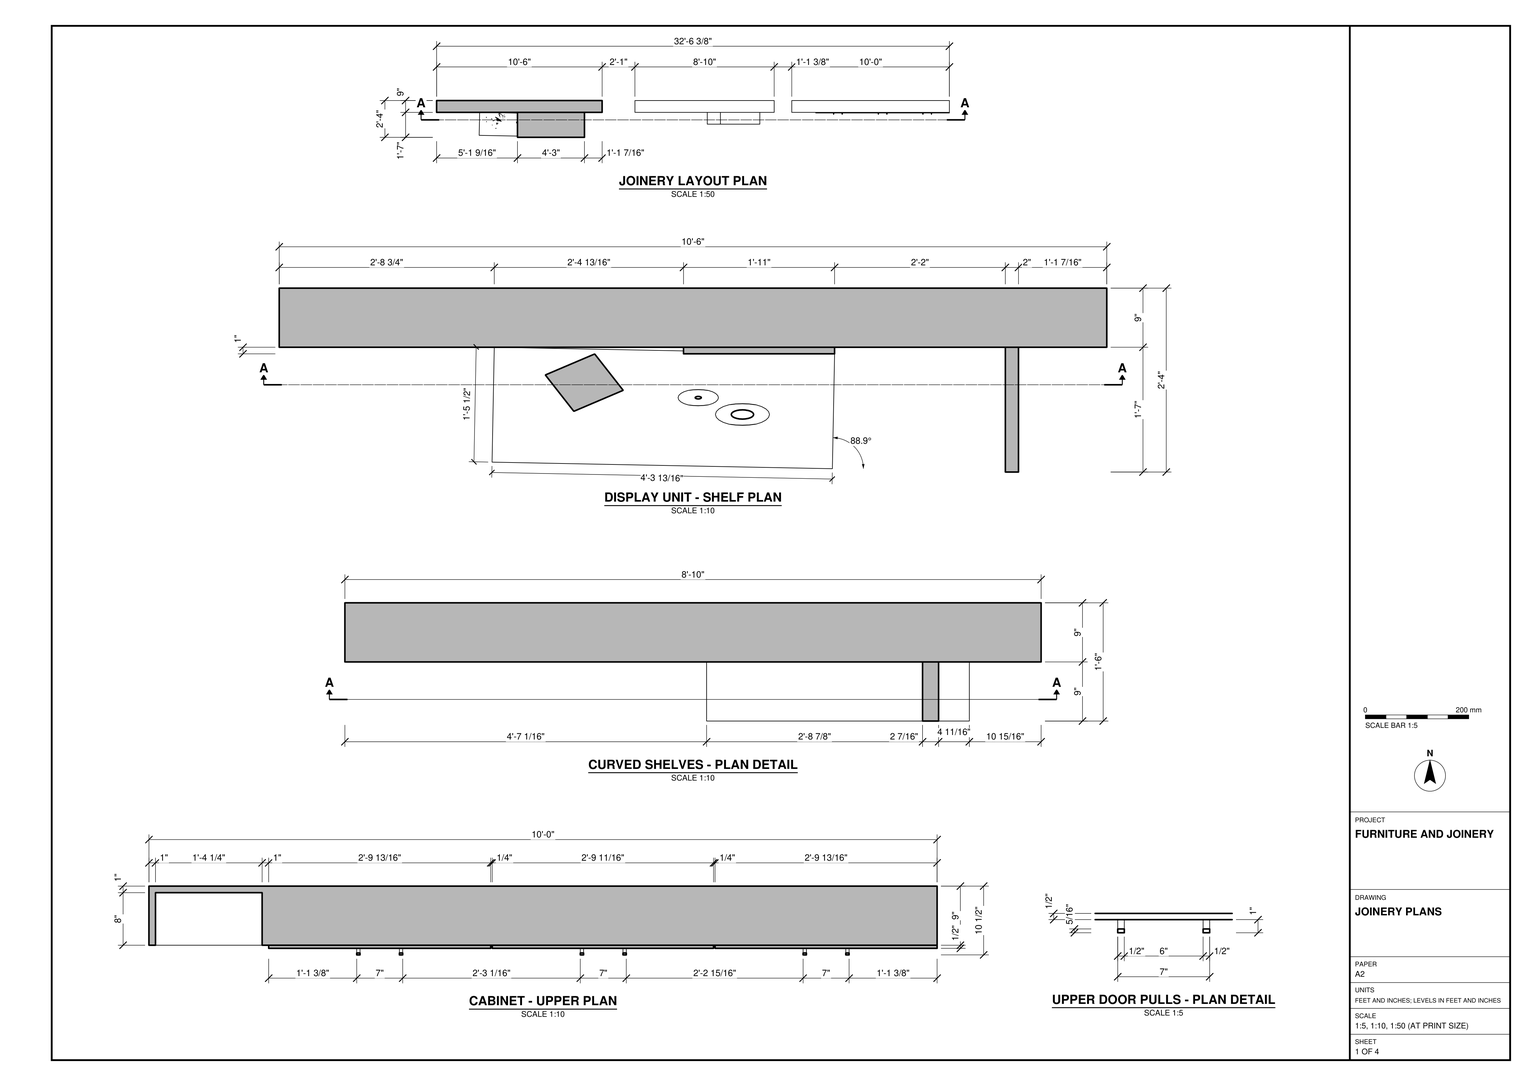
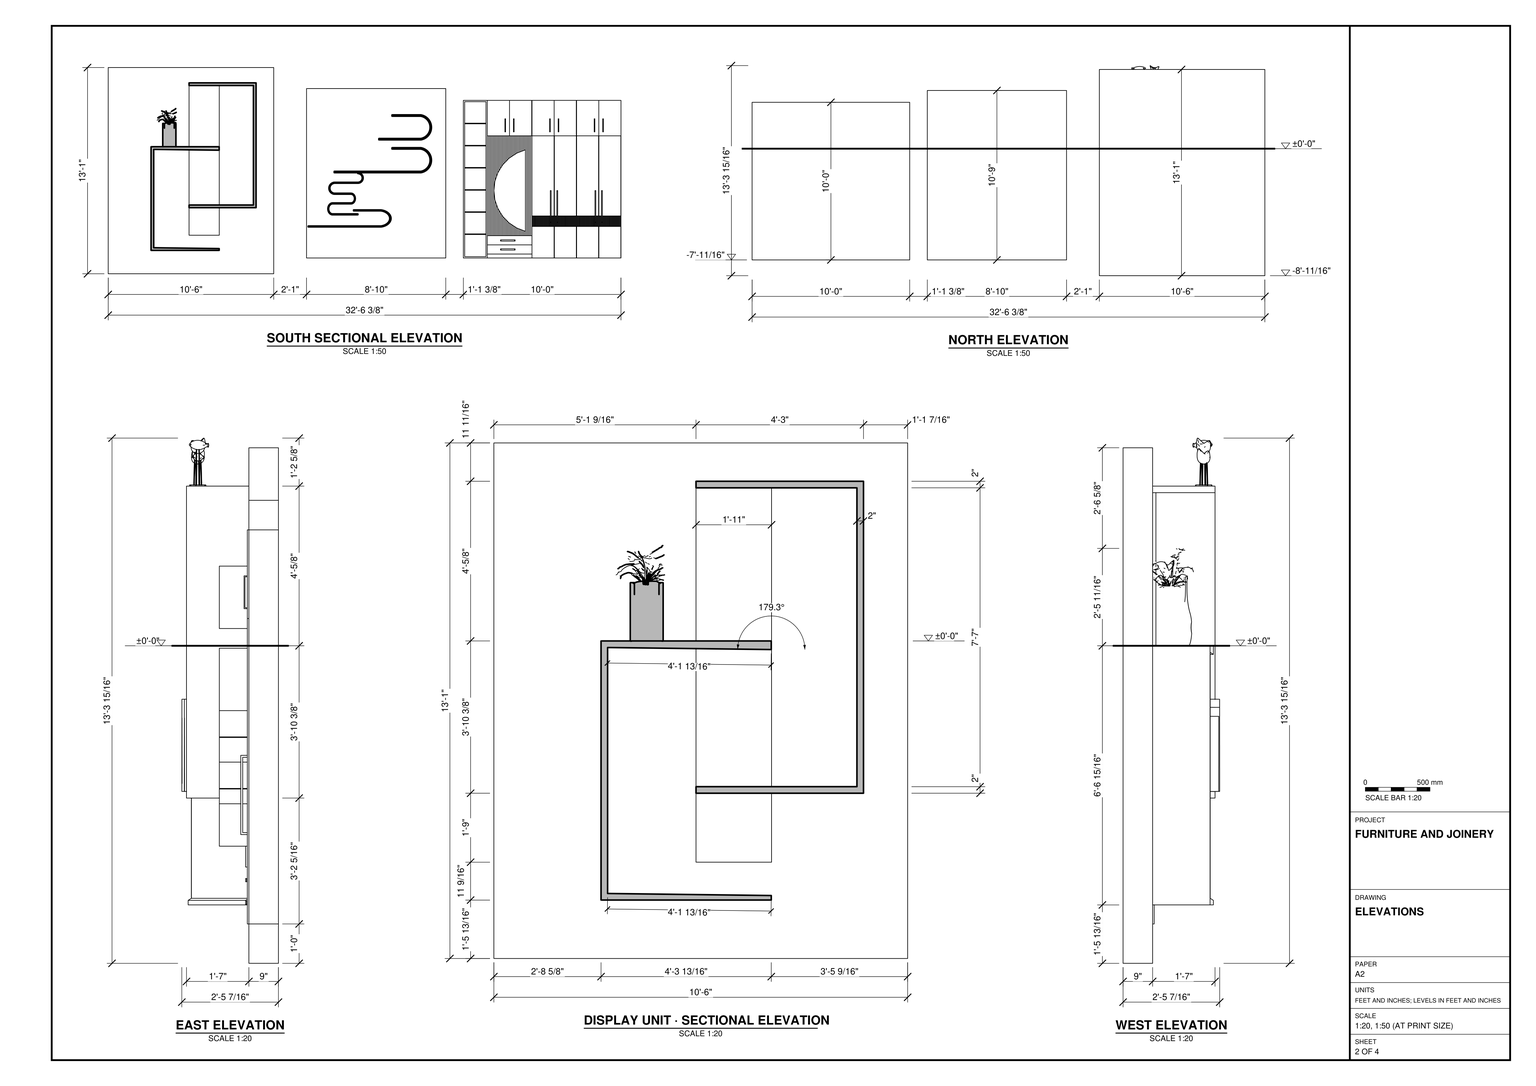
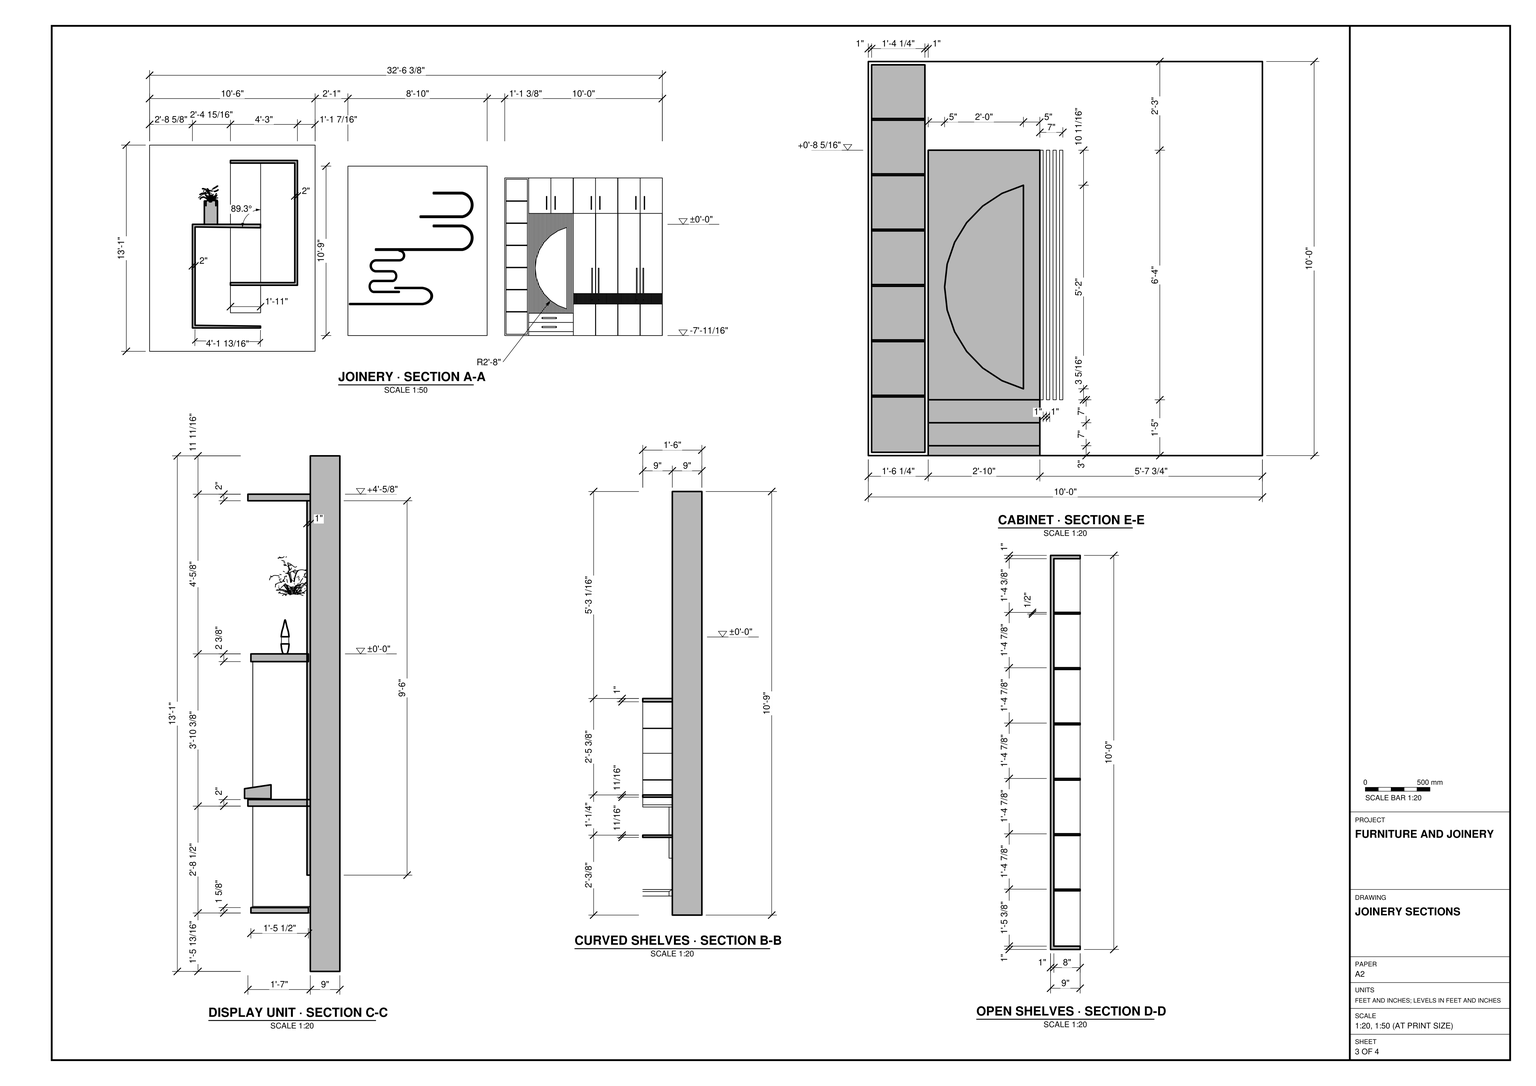
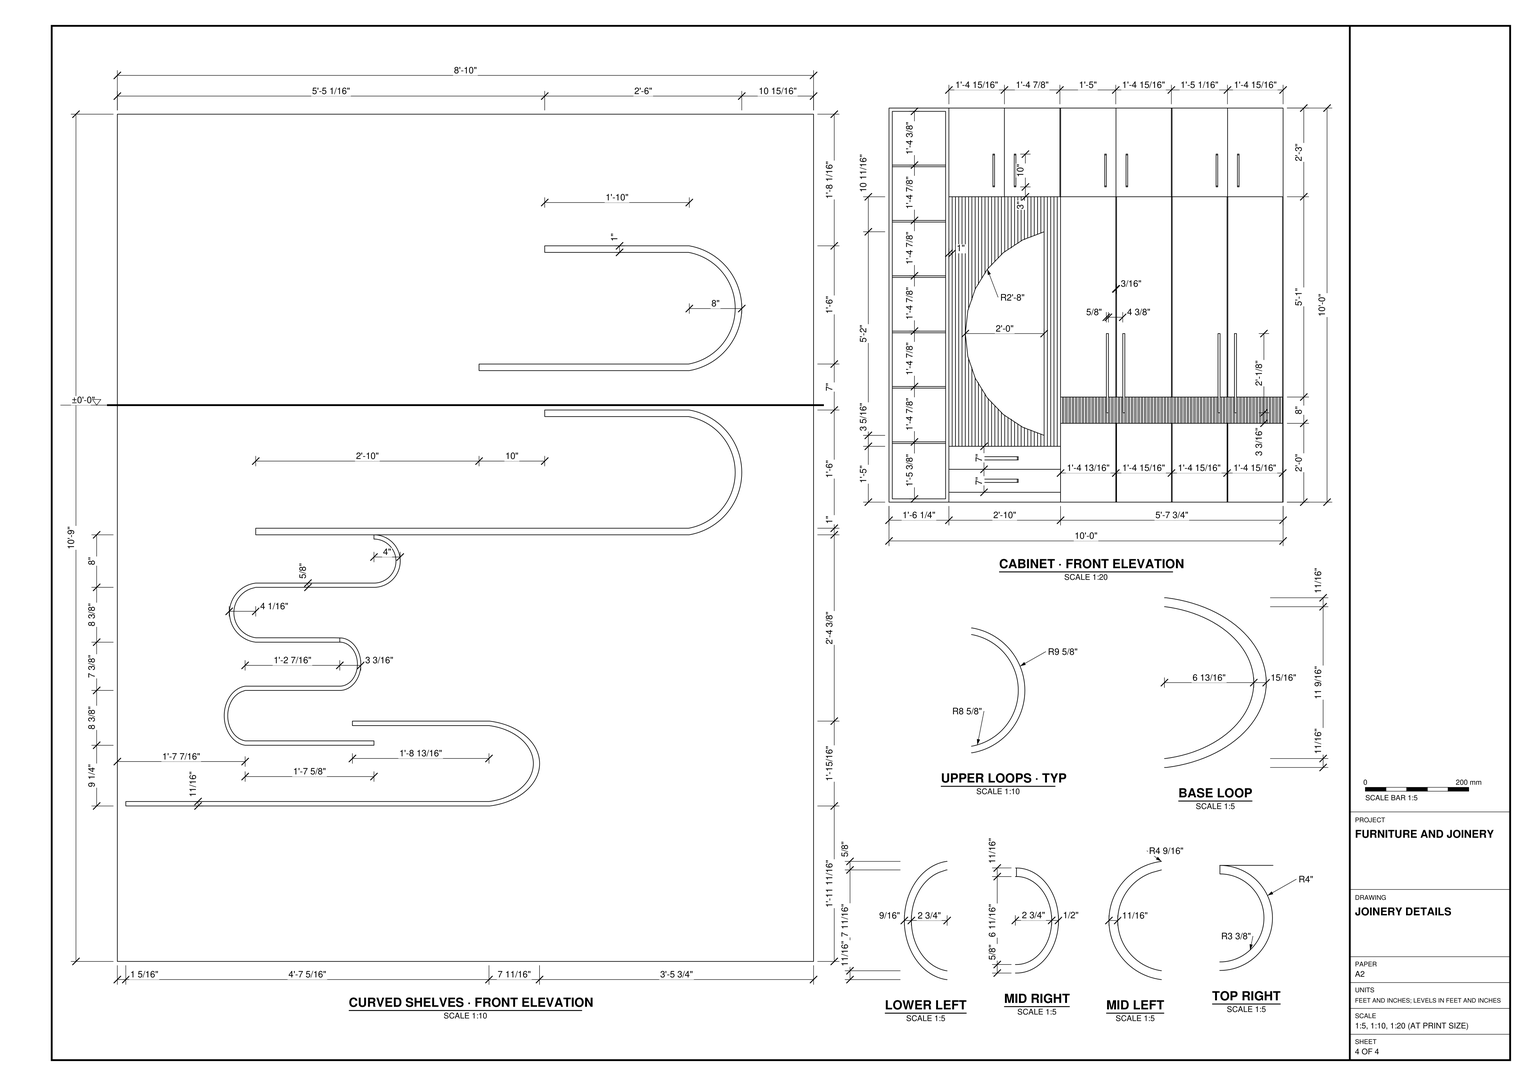
Build the three joinery pieces in SketchUp from task_files/diagram_01.pdf. Work in feet and inches. The complete arrangement is 32'-6 3/8" wide, 2'-5 7/16" deep and 13'-3 15/16" high. Use ±0'-0" as the common elevation datum, not as the bottom of the units.

Follow the south elevation from left to right: the framed display unit, the curved shelves and the storage cabinet. Align their backs in plan and leave the gaps dimensioned on the layout sheet. On the display unit, model the 9" thick backing panel and the projecting shelves with their vertical returns. The lower frame opens to the right and the upper frame opens to the left. On the middle unit, follow the horizontal shelf runs and rounded returns as they rise from the lower left to the upper right. Use the sections to set the shelf projections from the backing panels.

Build the cabinet with a full-height column of open shelves at the left, a recessed display bay with a semicircular feature above two drawers, and closed storage at the right. Include the upper doors, lower fronts and projecting pulls shown in the drawings. Decor and loose items may be any suitable library components placed as shown. Keep each joinery piece in a separate group or component and use components for repeated parts. Save one SketchUp model as output_files/display_unit_curved_shelves_and_storage_cabinet.skp.

# SketchUp Ruby script. Lengths in inches.
U = 1.inch
M = Sketchup.active_model
def pt(a) = Geom::Point3d.new(a.map { |v| v * U })
def face(e, loops, mat)
  f = e.add_face(loops[0].map { |a| pt(a) })
  loops[1..].each { |l| e.add_face(l.map { |a| pt(a) }).erase! }
  f.material = f.back_material = mat if mat
  f
end
# faces: each face lists its corners as indices into pts; further lists are holes
def faces(e, pts, list, mat = nil) = list.each { |f| face(e, (f[0].is_a?(Array) ? f : [f]).map { |l| l.map { |i| pts[i] } }, mat) }
# xy, xz, yz: faces in a plane at the given z, y or x. An outline is a flat list of corners, or four numbers for a rectangle; further outlines are holes
def ring(l) = l.size == 4 ? [[l[0], l[1]], [l[2], l[1]], [l[2], l[3]], [l[0], l[3]]] : l.each_slice(2).to_a
def flat(e, list, mat, &to3) = list.each { |f| face(e, (f[0].is_a?(Array) ? f : [f]).map { |l| ring(l).map { |u, v| to3.(u, v) } }, mat) }
def xy(e, z, list, mat = nil) = flat(e, list, mat) { |x, y| [x, y, z] }
def xz(e, y, list, mat = nil) = flat(e, list, mat) { |x, z| [x, y, z] }
def yz(e, x, list, mat = nil) = flat(e, list, mat) { |y, z| [x, y, z] }
def lines(e, pts, list) = list.each { |a, b| e.add_line(pt(pts[a]), pt(pts[b])) }
# prism: a flat outline (further loops are holes) pulled along v
def prism(e, loops, v, mat = nil)
  f = face(e, loops, mat); d = Geom::Vector3d.new(v.map { |x| x * U })
  f.pushpull(f.normal.samedirection?(d) ? d.length : -d.length)
end
def box(e, o, s, mat = nil) = prism(e, [[o, [o[0] + s[0], o[1], o[2]], [o[0] + s[0], o[1] + s[1], o[2]], [o[0], o[1] + s[1], o[2]]]], [0, 0, s[2]], mat)
def at(x, y, z, deg = 0) = Geom::Transformation.translation(pt([x, y, z])) * Geom::Transformation.rotation(ORIGIN, Z_AXIS, deg.degrees)
def axes(o, x, y, z) = Geom::Transformation.new([*x, 0, *y, 0, *z, 0, *pt(o).to_a, 1])
def part(name) = M.definitions.add(name)
# library, detail: a bought-in or finely detailed component or shape, given as its bounding box
def library(name, o, s) = part(name).tap { |d| box(d.entities, o, s) }
def detail(e, o, s) = box(e.add_group.entities, o, s)
def put(e, d, t, mat = nil) = e.add_instance(d, t).tap { |i| i.material = mat if mat }
def group(e, t, mat = nil) = e.add_group.tap { |g| g.transformation = t; g.material = mat if mat }.entities
root = M.entities
M.materials.add("[Color A01]").color = [101, 116, 79]
M.materials.add("[Color A01]1").color = [196, 189, 165]
M.materials.add("[Color A01]2").color = [176, 132, 93]
M.materials.add("[Color A02]").color = [127, 133, 94]
M.materials.add("[Color C02]").color = [255, 204, 153]
M.materials.add("[Color M09]").color = [0, 0, 0]
M.materials.add("[Wood Cherry Original]").color = [152, 86, 42]
c1 = library("Untitled",[0,0,0],[7.78,10.125,9.38])
c2 = library("Ceramic Birds on",[-120.01,56.07,-27.09],[117.74,27.05,54.18])
c3 = library("SimLab\#1",[-237.64,52,0],[43.92,43.98,50.37])
c4 = part("Vertical wood slat")
box(c4.entities,[0,-2,0],[1,2,76],"[Wood Cherry Original]")
c5 = part("Group\#7")
prism(c5.entities,[[[0.625,2,0],[0.625,2,0.59],[0.625,0.59,0.59],[0.625,0.59,23.53],[0.625,2,23.53],[0.625,2,24.13],[0.625,0,24.13],[0.625,0,0]]],[-0.625,0,0])
c6 = part("Group\#5")
prism(c6.entities,[[[0.5,1,9.71],[0.5,1,10],[0.5,0,10],[0.5,0,0],[0.5,1,0],[0.5,1,0.29],[0.5,0.29,0.29],[0.5,0.29,9.71]]],[-0.5,0,0])
c7 = library("Group\#37",[208.35,-82.82,84.7],[13.92,5.45,20.99])
xy(root,5.8,[[84.22,0.51,32.41,1.51,32.74,19,84.56,18]],"[Color A01]2")
xy(root,84.7,[[84.22,0.51,84.56,18,32.74,19,32.41,1.51]],"[Color A01]2")
p = [[84.22,0.51,5.8],[84.22,0.51,7.18],[34.4,1.47,7.8],[34.4,1.47,82.7],[84.22,0.51,82.08],[84.22,0.51,84.7],
  [32.41,1.51,84.7],[32.41,1.51,5.8],[84.56,18,5.8],[84.56,18,7.18],[32.74,19,84.7],[32.74,19,5.8],
  [84.56,18,84.7],[84.56,18,82.08],[34.74,18.96,82.7],[34.74,18.96,7.8]]
faces(root,p,[[0,1,2,3,4,5,6,7],[10,11,7,6],[3,2,15,14],[4,3,14,13],[4,13,12,5]],"[Color A01]2")
faces(root,p,[[8,9,1,0],[12,13,14,15,9,8,11,10]])
put(root,c1,axes([110.34,0.03,40.32],[-0.12671,1.68524,0],[-4.76654,-0.3584,0],[0,0,3]))
put(root,c2,axes([102.2,-15.7,140.64],[0.23902,0,0],[0,0.28,0],[0,0,0.2698]))
put(root,c3,axes([171.33,-17.61,84.65],[0.58,0,0],[0,0.4272,0],[0,0,0.59]))
g1 = group(root,at(270.37,16.53,0))
prism(g1,[[[39.05,2.47,12.84],[39.35,2.47,12.84],[39.35,1.47,12.84],[28.35,1.47,12.84],[28.35,2.47,12.84],[28.65,2.47,12.84],[28.65,1.77,12.84],[39.05,1.77,12.84]]],[0,0,1],"[Color M09]")
prism(g1,[[[39.05,2.47,6],[39.35,2.47,6],[39.35,1.47,6],[28.35,1.47,6],[28.35,2.47,6],[28.65,2.47,6],[28.65,1.77,6],[39.05,1.77,6]]],[0,0,1],"[Color M09]")
put(g1,c4,at(34.23,10.47,17))
put(g1,c4,at(24.23,10.47,17))
put(g1,c4,at(46.23,10.47,17))
put(g1,c4,at(48.23,10.47,17))
put(g1,c4,at(44.23,10.47,17))
put(g1,c4,at(18.23,10.47,17))
put(g1,c4,at(20.23,10.47,17))
put(g1,c4,at(26.23,10.47,17))
put(g1,c4,at(42.23,10.47,17))
put(g1,c4,at(28.23,10.47,17))
put(g1,c4,at(36.23,10.47,17))
put(g1,c4,at(30.23,10.47,17))
put(g1,c4,at(22.23,10.47,17))
put(g1,c4,at(32.23,10.47,17))
put(g1,c4,at(38.23,10.47,17))
put(g1,c4,at(40.23,10.47,17))
put(g1,c4,at(50.23,10.47,17))
put(g1,c4,at(54.23,10.47,17))
put(g1,c4,at(58.23,10.47,17))
put(g1,c4,at(52.23,10.47,17))
put(g1,c4,at(56.23,10.47,17))
g2 = group(g1,at(23.23,8.39,20.33))
xz(g2,0,[[[24,0,17.44,2.49,11.58,6.35,6.7,11.4,3.04,17.38,0.77,24.02,0,31,0.77,37.98,3.04,44.62,6.7,50.6,11.58,55.65,17.44,59.51,24,62],[21.5,3.63,21.5,58.37,18.59,57.27,13.1875,53.71,8.69,49.06,5.32,43.54,3.23,37.43,2.52,31,3.23,24.57,5.32,18.46,8.69,12.94,13.1875,8.29,18.59,4.73]]])
g3 = group(g1,at(23.23,6.31,20.33))
xz(g3,0,[[24,0,24,62,17.44,59.51,11.58,55.65,6.7,50.6,3.04,44.62,0.77,37.98,0,31,0.77,24.02,3.04,17.38,6.7,11.4,11.58,6.35,17.44,2.49]])
xz(g3,2,[[[24,0,17.44,2.49,11.58,6.35,6.7,11.4,3.04,17.38,0.77,24.02,0,31,0.77,37.98,3.04,44.62,6.7,50.6,11.58,55.65,17.44,59.51,24,62],[21.5,3.63,21.5,58.37,18.59,57.27,13.1875,53.71,8.69,49.06,5.32,43.54,3.23,37.43,2.52,31,3.23,24.57,5.32,18.46,8.69,12.94,13.1875,8.29,18.59,4.73]],[21.5,3.63,18.59,4.73,13.1875,8.29,8.69,12.94,5.32,18.46,3.23,24.57,2.52,31,3.23,37.43,5.32,43.54,8.69,49.06,13.1875,53.71,18.59,57.27,21.5,58.37]])
yz(g3,24,[[0,0,2,62]])
p = [[24,0,0],[17.44,0,2.49],[17.44,2,2.49],[24,2,0],[11.58,0,6.35],[11.58,2,6.35],
  [6.7,0,11.4],[6.7,2,11.4],[3.04,0,17.38],[3.04,2,17.38],[0.77,0,24.02],[0.77,2,24.02],
  [0,0,31],[0,2,31],[0.77,0,37.98],[0.77,2,37.98],[3.04,0,44.62],[3.04,2,44.62],
  [6.7,0,50.6],[6.7,2,50.6],[11.58,0,55.65],[11.58,2,55.65],[17.44,0,59.51],[17.44,2,59.51],
  [24,0,62],[24,2,62]]
faces(g3,p,[[0,1,2,3],[1,4,5,2],[4,6,7,5],[6,8,9,7],[8,10,11,9],[10,12,13,11],[12,14,15,13],[14,16,17,15],
  [16,18,19,17],[18,20,21,19],[20,22,23,21],[22,24,25,23]])
g4 = group(g1,at(0,2.47,0),"[Color A01]")
xy(g4,0,[[52.232,-0.472,69.056,0],[69.295,-0.472,85.998,0],[86.234,-0.472,102.94,0],[103.176,-0.472,119.882,0],[0,0,0,9,120,9,120,0,52.232,0,52.232,8,18.232,8,18.232,0]])
xy(g4,1,[[1,0,17.232,8]])
xy(g4,17.857,[[1,0,17.232,8]])
xy(g4,18.357,[[1,0,17.232,8]])
xy(g4,34.714,[[1,0,17.232,8]])
xy(g4,35.214,[[1,0,17.232,8]])
xy(g4,51.571,[[1,0,17.232,8]])
xy(g4,52.071,[[1,0,17.232,8]])
xy(g4,68.429,[[1,0,17.232,8]])
xy(g4,68.929,[[1,0,17.232,8]])
xy(g4,85.286,[[1,0,17.232,8]])
xy(g4,85.786,[[1,0,17.232,8]])
xy(g4,93,[[18.232,-0.472,52.037,0],[52.232,-0.472,52.273,0],[52.273,-0.472,69.056,0],[69.056,-0.472,69.295,0],[69.295,-0.472,85.959,0],
  [85.959,-0.472,85.998,0],[86.196,-0.472,86.234,0],[86.234,-0.472,102.94,0],[102.94,-0.472,103.176,0],[103.176,-0.472,119.882,0],
  [119.882,-0.472,120,0],[18.232,0,52.037,8],[52.037,0,52.155,8],[52.155,0,52.232,8]])
xy(g4,102.143,[[1,0,17.232,8]])
xy(g4,102.643,[[1,0,17.232,8]])
xy(g4,119,[[1,0,17.232,8]])
xy(g4,120,[[18.232,-0.472,52.037,0],[52.273,-0.472,85.959,0],[86.196,-0.472,120,0],[0,0,120,9]])
xz(g4,-0.472,[[52.81,24,53.232,32],[53.81,24,54.232,32],[54.81,24,55.232,32],[55.81,24,56.232,32],[56.81,24,57.232,32],
  [57.81,24,58.232,32],[58.81,24,59.232,32],[59.81,24,60.232,32],[60.81,24,61.232,32],[61.81,24,62.232,32],
  [62.81,24,63.232,32],[63.81,24,64.232,32],[64.81,24,65.232,32],[65.81,24,66.232,32],[66.81,24,67.232,32],
  [67.81,24,68.232,32],[68.81,24,69.232,32],[69.81,24,70.232,32],[70.81,24,71.232,32],[71.81,24,72.232,32],
  [72.81,24,73.232,32],[73.81,24,74.232,32],[74.81,24,75.232,32],[75.81,24,76.232,32],[76.81,24,77.232,32],
  [77.81,24,78.232,32],[78.81,24,79.232,32],[79.81,24,80.232,32],[80.81,24,81.232,32],[81.81,24,82.232,32],
  [82.81,24,83.232,32],[83.81,24,84.232,32],[84.81,24,85.232,32],[85.81,24,86.232,32],[86.81,24,87.232,32],
  [87.81,24,88.232,32],[88.81,24,89.232,32],[89.81,24,90.232,32],[90.81,24,91.232,32],[91.81,24,92.232,32],
  [92.81,24,93.232,32],[93.81,24,94.232,32],[94.81,24,95.232,32],[95.81,24,96.232,32],[96.81,24,97.232,32],
  [97.81,24,98.232,32],[98.81,24,99.232,32],[99.81,24,100.232,32],[100.81,24,101.232,32],[101.81,24,102.232,32],
  [102.81,24,103.232,32],[103.81,24,104.232,32],[104.81,24,105.232,32],[105.81,24,106.232,32],[106.81,24,107.232,32],
  [107.81,24,108.232,32],[108.81,24,109.232,32],[109.81,24,110.232,32],[110.81,24,111.232,32],[111.81,24,112.232,32],
  [112.81,24,113.232,32],[113.81,24,114.232,32],[114.81,24,115.232,32],[115.81,24,116.232,32],[116.81,24,117.232,32],
  [117.81,24,118.232,32],[118.81,24,119.232,32],[119.81,24,119.882,32],[69.056,32,69.295,93],[102.94,32,103.176,93]])
xz(g4,-0.472,[[52.232,24,52.81,32],[53.232,24,53.81,32],[54.232,24,54.81,32],[55.232,24,55.81,32],[56.232,24,56.81,32],
  [57.232,24,57.81,32],[58.232,24,58.81,32],[59.232,24,59.81,32],[60.232,24,60.81,32],[61.232,24,61.81,32],
  [62.232,24,62.81,32],[63.232,24,63.81,32],[64.232,24,64.81,32],[65.232,24,65.81,32],[66.232,24,66.81,32],
  [67.232,24,67.81,32],[68.232,24,68.81,32],[69.232,24,69.81,32],[70.232,24,70.81,32],[71.232,24,71.81,32],
  [72.232,24,72.81,32],[73.232,24,73.81,32],[74.232,24,74.81,32],[75.232,24,75.81,32],[76.232,24,76.81,32],
  [77.232,24,77.81,32],[78.232,24,78.81,32],[79.232,24,79.81,32],[80.232,24,80.81,32],[81.232,24,81.81,32],
  [82.232,24,82.81,32],[83.232,24,83.81,32],[84.232,24,84.81,32],[85.232,24,85.81,32],[86.232,24,86.81,32],
  [87.232,24,87.81,32],[88.232,24,88.81,32],[89.232,24,89.81,32],[90.232,24,90.81,32],[91.232,24,91.81,32],
  [92.232,24,92.81,32],[93.232,24,93.81,32],[94.232,24,94.81,32],[95.232,24,95.81,32],[96.232,24,96.81,32],
  [97.232,24,97.81,32],[98.232,24,98.81,32],[99.232,24,99.81,32],[100.232,24,100.81,32],[101.232,24,101.81,32],
  [102.232,24,102.81,32],[103.232,24,103.81,32],[104.232,24,104.81,32],[105.232,24,105.81,32],[106.232,24,106.81,32],
  [107.232,24,107.81,32],[108.232,24,108.81,32],[109.232,24,109.81,32],[110.232,24,110.81,32],[111.232,24,111.81,32],
  [112.232,24,112.81,32],[113.232,24,113.81,32],[114.232,24,114.81,32],[115.232,24,115.81,32],[116.232,24,116.81,32],
  [117.232,24,117.81,32],[118.232,24,118.81,32],[119.232,24,119.81,32],[18.232,93,35.135,120],[35.135,93,52.037,120],
  [52.273,93,69.116,120],[69.116,93,85.959,120],[86.196,93,103.098,120],[103.098,93,120,120]],"[Color A01]")
xz(g4,-0.472,[[52.232,0,69.056,24],[69.295,0,85.998,24],[86.234,0,102.94,24],[103.176,0,119.882,24],[52.232,32,69.056,93],
  [69.295,32,85.998,93],[86.234,32,102.94,93],[103.176,32,119.882,93]],"[Color A01]1")
xz(g4,0,[[[0,0,18.232,120],[1,1,17.232,119]],[52.232,0,69.056,93],[69.056,0,69.174,93],[69.174,0,69.295,93],[69.295,0,85.998,93],
  [85.998,0,86.234,93],[86.234,0,102.94,93],[102.94,0,103.058,93],[103.058,0,103.176,93],[103.176,0,119.882,93],
  [119.882,0,120,93],[1,17.857,17.232,18.357],[1,34.714,17.232,35.214],[1,51.571,17.232,52.071],[1,68.429,17.232,68.929],
  [1,85.286,17.232,85.786],[18.232,93,52.037,120],[52.037,93,52.273,120],[52.273,93,85.959,120],[85.959,93,86.196,120],
  [86.196,93,120,120],[1,102.143,17.232,102.643]])
xz(g4,8,[[18.232,0,52.232,93],[1,1,17.232,18.357],[1,18.357,17.232,35.214],[1,35.214,17.232,52.071],[1,52.071,17.232,68.929],
  [1,68.929,17.232,85.786],[1,85.786,17.232,102.643],[1,102.643,17.232,119]])
xz(g4,9,[[0,0,120,120]])
yz(g4,0,[[0,0,9,120]])
yz(g4,1,[[0,1,8,18.357],[0,18.357,8,35.214],[0,35.214,8,52.071],[0,52.071,8,68.929],[0,68.929,8,85.786],
  [0,85.786,8,102.643],[0,102.643,8,119]])
yz(g4,17.232,[[0,1,8,18.357],[0,18.357,8,35.214],[0,35.214,8,52.071],[0,52.071,8,68.929],[0,68.929,8,85.786],
  [0,85.786,8,102.643],[0,102.643,8,119]])
yz(g4,18.232,[[0,0,8,93],[-0.472,93,0,120]])
yz(g4,52.037,[[-0.472,93,0,120]])
yz(g4,52.232,[[-0.472,0,0,93],[0,0,8,93]])
yz(g4,52.273,[[-0.472,93,0,120]])
yz(g4,85.959,[[-0.472,93,0,120]])
yz(g4,86.196,[[-0.472,93,0,120]])
yz(g4,119.882,[[-0.472,0,0,93]])
yz(g4,120,[[0,0,9,120],[-0.472,93,0,120]])
g5 = group(g1,at(18.23,2.47,0),"[Color A01]")
xy(g5,0,[[0,2,34,8]])
xy(g5,3,[[0,0,34,2],[0,2,34,8]])
xy(g5,10,[[0,0,34,8]])
xy(g5,17,[[0,0,34,8]])
xz(g5,0,[[0,3,34,10],[0,10,34,17]])
xz(g5,2,[[0,0,34,3]])
xz(g5,8,[[0,0,34,3],[0,3,34,10],[0,10,34,17]])
yz(g5,0,[[2,0,8,3],[0,3,8,10],[0,10,8,17]])
yz(g5,34,[[2,0,8,3],[0,3,8,10],[0,10,8,17]])
put(g1,c5,at(105.1875,0,27.21),"[Color M09]")
g6 = group(g1,at(66.1875,0,27.21),"[Color M09]")
prism(g6,[[[0.625,2,0],[0.625,2,0.59],[0.625,0.59,0.59],[0.625,0.59,23.53],[0.625,2,23.53],[0.625,2,24.13],[0.625,0,24.13],[0.625,0,0]]],[-0.625,0,0])
put(g1,c5,at(71.1875,0,27.21),"[Color M09]")
put(g1,c5,at(100.1875,0,27.21),"[Color M09]")
put(g1,c6,at(38.13,1,96),"[Color M09]")
put(g1,c6,at(65.68,1,96),"[Color M09]")
put(g1,c6,at(99.6,1,96),"[Color M09]")
put(g1,c6,at(72.18,1,96),"[Color M09]")
put(g1,c6,at(106.1,1,96),"[Color M09]")
put(g1,c6,at(31.63,1,96),"[Color M09]")
g7 = group(root,at(150.98,10,0))
detail(g7,[55.07,0,89.96],[40,9,19])
detail(g7,[16.27,0,32.91],[78.8,9,51.05])
detail(g7,[1.29,0,23.67],[63,9,12.92])
g8 = group(g7,at(0,9,6),"[Color C02]")
box(g8,[0,0,-6],[106,9,129])
g9 = group(root,at(0,19,0),"[Color A02]")
box(g9,[0,0,-12],[126,9,157])
g10 = group(root,at(61.56,0,38.33),"[Color A01]2")
prism(g10,[[[0,0,95],[0,0,93],[49,0,93],[49,0,2],[0,0,2],[0,0,0],[51,0,0],[51,0,95]]],[0,19,0])
g11 = group(root,at(61.56,18,17.33),"[Color A01]2")
box(g11,[0,0,0],[23,1,114])
g12 = group(root,at(34.4,0.51,7.18),"[Color A01]2")
p = [[0,0.96,0.62],[49.8125,0,0],[50.15,17.49,0],[0.34,18.45,0.62]]
faces(g12,p,[[0,1,2,3]])
put(root,c7,at(-147.63,89.93,0))
